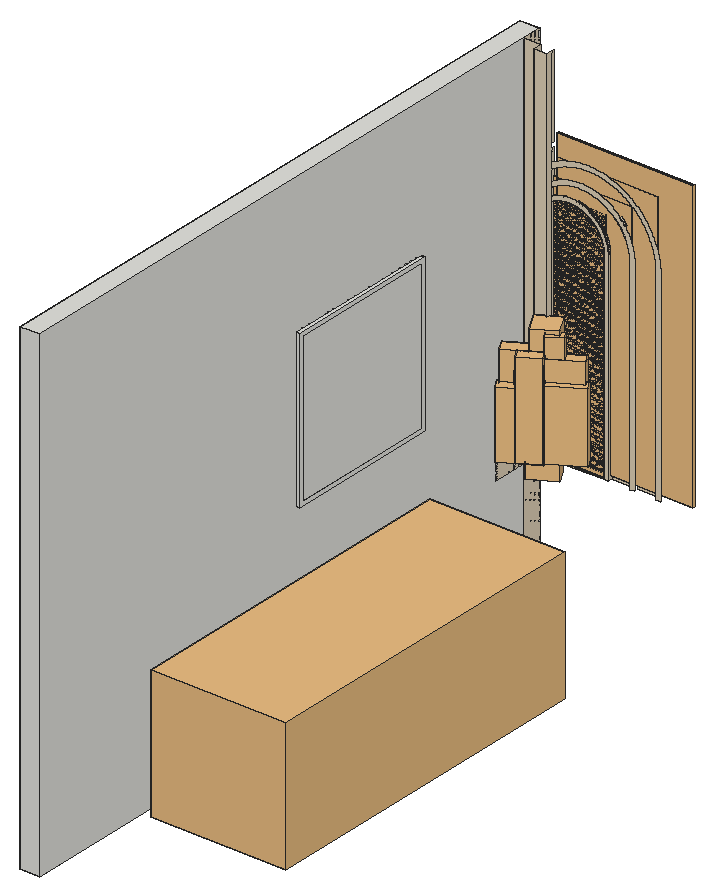
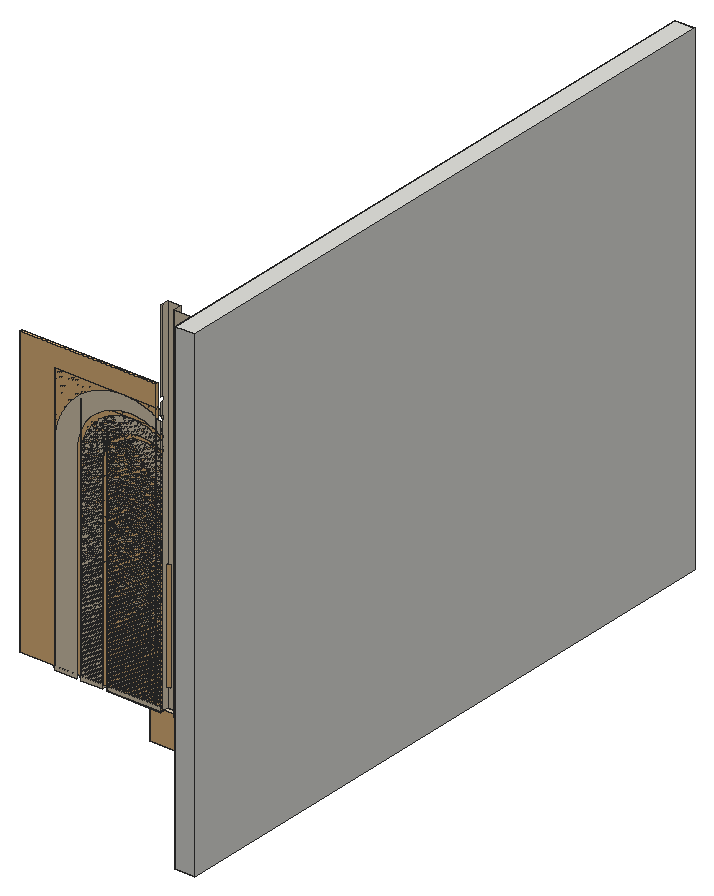
# SketchUp Ruby script. Lengths in inches.
U = 1.inch
M = Sketchup.active_model
def pt(a) = Geom::Point3d.new(a.map { |v| v * U })
def face(e, loops, mat)
  f = e.add_face(loops[0].map { |a| pt(a) })
  loops[1..].each { |l| e.add_face(l.map { |a| pt(a) }).erase! }
  f.material = f.back_material = mat if mat
  f
end
# faces: each face lists its corners as indices into pts; further lists are holes
def faces(e, pts, list, mat = nil) = list.each { |f| face(e, (f[0].is_a?(Array) ? f : [f]).map { |l| l.map { |i| pts[i] } }, mat) }
# xy, xz, yz: faces in a plane at the given z, y or x. An outline is a flat list of corners, or four numbers for a rectangle; further outlines are holes
def ring(l) = l.size == 4 ? [[l[0], l[1]], [l[2], l[1]], [l[2], l[3]], [l[0], l[3]]] : l.each_slice(2).to_a
def flat(e, list, mat, &to3) = list.each { |f| face(e, (f[0].is_a?(Array) ? f : [f]).map { |l| ring(l).map { |u, v| to3.(u, v) } }, mat) }
def xy(e, z, list, mat = nil) = flat(e, list, mat) { |x, y| [x, y, z] }
def xz(e, y, list, mat = nil) = flat(e, list, mat) { |x, z| [x, y, z] }
def yz(e, x, list, mat = nil) = flat(e, list, mat) { |y, z| [x, y, z] }
def lines(e, pts, list) = list.each { |a, b| e.add_line(pt(pts[a]), pt(pts[b])) }
# prism: a flat outline (further loops are holes) pulled along v
def prism(e, loops, v, mat = nil)
  f = face(e, loops, mat); d = Geom::Vector3d.new(v.map { |x| x * U })
  f.pushpull(f.normal.samedirection?(d) ? d.length : -d.length)
end
def box(e, o, s, mat = nil) = prism(e, [[o, [o[0] + s[0], o[1], o[2]], [o[0] + s[0], o[1] + s[1], o[2]], [o[0], o[1] + s[1], o[2]]]], [0, 0, s[2]], mat)
def at(x, y, z, deg = 0) = Geom::Transformation.translation(pt([x, y, z])) * Geom::Transformation.rotation(ORIGIN, Z_AXIS, deg.degrees)
def axes(o, x, y, z) = Geom::Transformation.new([*x, 0, *y, 0, *z, 0, *pt(o).to_a, 1])
def part(name) = M.definitions.add(name)
# library, detail: a bought-in or finely detailed component or shape, given as its bounding box
def library(name, o, s) = part(name).tap { |d| box(d.entities, o, s) }
def detail(e, o, s) = box(e.add_group.entities, o, s)
def put(e, d, t, mat = nil) = e.add_instance(d, t).tap { |i| i.material = mat if mat }
def group(e, t, mat = nil) = e.add_group.tap { |g| g.transformation = t; g.material = mat if mat }.entities
root = M.entities
M.materials.add("POT_TEXTURE_1").color = [172, 172, 172]
M.materials.add("Teddy_Brim").color = [225, 210, 185]
M.materials.add("soil1").color = [68, 55, 47]
c1 = library("Group\#92",[-662.41,217.3,320.04],[397.32,658.3,1732.06])
c2 = library("Group\#94",[-299.2,181.55,262.58],[360.65,735.71,1258.34])
c3 = library("Group\#89",[-1038.76,656.55,345.34],[733.18,460.51,2065.7])
c4 = library("Group\#87",[-445.29,890.31,329.28],[284.3,304.08,2023.29])
c5 = library("Group\#90",[-733.48,439.625,202.64],[456.28,533.12,1536.78])
c6 = library("Group\#93",[-455.56,899.32,410.78],[341.21,610.33,1581.5])
c7 = library("Group\#86",[-516.34,626.77,-4.5625],[517.73,515.95,418.98])
c8 = library("Group\#91",[-249.24,914.85,310.18],[345.55,647.95,1307.93])
c9 = library("Group\#88",[-277.97,488.68,287.26],[362.84,405.94,1768.54])
c10 = library("Group\#85",[-468.76,669.89,380.1875],[424.36,427.47,41.99])
c11 = part("Potted plant")
put(c11.entities,c1,at(1038.76,-181.55,4.5625))
put(c11.entities,c2,at(1038.76,-181.55,4.5625))
put(c11.entities,c3,at(1038.76,-181.55,4.5625))
put(c11.entities,c4,at(1038.76,-181.55,4.5625))
put(c11.entities,c5,at(1038.76,-181.55,4.5625))
put(c11.entities,c6,at(1038.76,-181.55,4.5625))
put(c11.entities,c7,at(1038.76,-181.55,4.5625),"POT_TEXTURE_1")
put(c11.entities,c8,at(1038.76,-181.55,4.5625))
put(c11.entities,c9,at(1038.76,-181.55,4.5625))
put(c11.entities,c10,at(1038.76,-181.55,4.5625),"soil1")
c12 = library("Group\#4",[0,0,0],[12.36,0.5,54.3])
c13 = library("Group\#3",[0,0,0],[18.36,0.5,57.11])
c14 = library("sofaD71839)",[0.35,-39.08,0.31],[80.46,34.29,30.24])
c15 = library("Group\#5",[0,0,0],[23.36,0.5,61.38])
c16 = library("Group\#155",[0,0,0],[31.36,0.5,66.36])
xy(root,34,[[8.5,137.5,11.5,137.6875],[8.5,137.6875,8.5,139.5,4.5,139.5,4.5,138.6875,11.5,138.6875,11.5,137.6875],[8.5,137.6875,11.5,138.6875],[11.5,138.5,23.86,138.6875],[23.86,138.5,24.86,138.6875],
  [11.5,138.6875,23.86,139.5]],"Teddy_Brim")
xy(root,88.29,[[15.22,138.5,15.4,139],[15.92,138.5,16.09,139]],"Teddy_Brim")
xy(root,88.3,[[15.57,138.5,15.74,139]],"Teddy_Brim")
xz(root,137.5,[[8.5,34,11.5,118]],"Teddy_Brim")
xz(root,138.5,[[11.5,33.76,11.5,34,24.86,34,24.86,80.61,24.85,80.8,24.85,80.98,24.83,81.17,24.82,81.35,24.8,81.54,24.77,81.72,24.75,81.9,24.72,82.08,24.68,82.27,24.64,82.45,24.6,82.625,24.55,82.81,24.5,82.98,24.45,83.16,24.39,83.34,24.33,83.51,24.26,83.68,24.19,83.86,24.12,84.03,24.05,84.19,23.97,84.36,23.88,84.53,23.8,84.69,23.71,84.85,23.61,85.01,23.52,85.17,23.42,85.33,23.3125,85.48,23.21,85.63,22.99,85.93,22.63,86.35,22.5,86.49,22.38,86.62,22.25,86.75,22.11,86.88,21.98,87.01,21.56,87.37,21.11,87.7,20.96,87.8,20.8,87.91,20.65,88,20.49,88.1,20.33,88.19,20.16,88.28,20,88.36,19.66,88.52,19.5,88.59,19.32,88.66,19.15,88.73,18.98,88.79,18.8,88.85,18.625,88.91,18.45,88.96,18.27,89.01,17.73,89.13,17.55,89.16,17.36,89.19,17.18,89.22,17,89.24,16.8125,89.26,16.63,89.27,16.44,89.28,16.26,89.28,16.07,89.29,15.89,89.28,15.7,89.28,15.52,89.27,15.33,89.26,14.97,89.22,14.78,89.19,14.42,89.13,14.06,89.05,13.875,89.01,13.7,88.96,13.52,88.91,13.34,88.85,13.17,88.79,12.99,88.73,12.48,88.52,12.3125,88.44,12.15,88.36,11.98,88.27,11.82,88.1875,11.66,88.09,11.5,88,11.5,87.17,11.6,87.23,11.75,87.3125,11.9,87.39,12.06,87.47,12.21,87.55,12.37,87.62,12.53,87.68,12.69,87.75,12.85,87.81,13.02,87.87,13.18,87.92,13.52,88.02,13.68,88.06,13.85,88.1,14.02,88.13,14.19,88.17,14.36,88.2,14.53,88.22,14.71,88.24,15.05,88.28,15.22,88.29,15.4,88.29,15.57,88.3,15.74,88.3,15.92,88.29,16.09,88.29,16.26,88.28,16.43,88.26,16.61,88.24,16.78,88.22,16.95,88.19,17.12,88.17,17.29,88.13,17.46,88.1,17.63,88.06,17.8,88.01,17.96,87.97,18.13,87.92,18.29,87.86,18.46,87.8,18.78,87.68,19.1,87.54,19.25,87.47,19.41,87.39,19.5625,87.31,19.71,87.22,19.86,87.14,20.01,87.05,20.16,86.95,20.3,86.86,20.58,86.66,20.86,86.44,21.12,86.22,21.25,86.1,21.5,85.86,21.62,85.74,21.73,85.61,21.85,85.48,21.96,85.35,22.07,85.21,22.18,85.08,22.28,84.9375,22.38,84.8,22.48,84.65,22.58,84.51,22.76,84.21,22.84,84.0625,22.93,83.91,23,83.76,23.08,83.6,23.22,83.28,23.29,83.125,23.35,82.96,23.47,82.64,23.57,82.3,23.61,82.14,23.73,81.63,23.79,81.29,23.83,80.95,23.85,80.77,23.86,80.6,23.86,34],[29.86,34,30.86,34,30.86,81.15,30.85,81.43,30.81,81.97,30.78,82.24,30.75,82.5,30.67,83.04,30.61,83.31,30.56,83.57,30.5,83.83,30.43,84.1,30.27,84.62,30.1875,84.87,30.1,85.13,29.9,85.63,29.79,85.88,29.68,86.125,29.56,86.37,29.43,86.61,29.31,86.85,29.17,87.09,28.89,87.55,28.74,87.77,28.58,88,28.42,88.21,28.26,88.43,27.92,88.85,27.74,89.05,27.56,89.26,26.99,89.83,26.79,90.02,26.58,90.19,26.375,90.37,26.17,90.54,25.95,90.71,25.73,90.87,25.29,91.17,25.06,91.32,24.83,91.46,24.59,91.6,24.36,91.73,24.12,91.85,23.87,91.97,23.63,92.09,23.38,92.2,23.13,92.3,22.875,92.4,22.62,92.49,22.37,92.58,21.85,92.74,21.59,92.81,21.32,92.87,21.06,92.93,20.79,92.98,20.53,93.03,19.99,93.11,19.72,93.13,19.45,93.16,19.18,93.18,18.91,93.1875,18.64,93.19,18.1,93.19,17.29,93.13,17.02,93.1,16.48,93.02,16.21,92.97,15.95,92.92,15.68,92.86,15.42,92.8,15.16,92.73,14.64,92.57,14.38,92.48,14.13,92.38,13.88,92.29,13.38,92.07,13.14,91.96,12.89,91.83,12.65,91.71,12.42,91.58,12.18,91.44,11.95,91.3,11.72,91.15,11.5,91,11.5,90.05,11.7,90.1875,11.92,90.33,12.36,90.59,12.58,90.71,12.8125,90.83,13.04,90.95,13.28,91.06,13.51,91.16,13.75,91.26,14.23,91.44,14.47,91.52,14.72,91.6,15.22,91.74,15.72,91.86,15.97,91.91,16.22,91.95,16.48,91.99,16.73,92.03,16.99,92.05,17.25,92.08,17.5,92.09,18.02,92.11,18.28,92.11,18.53,92.1,18.79,92.09,19.05,92.07,19.3,92.05,19.56,92.02,19.81,91.99,20.07,91.95,20.32,91.9,20.58,91.85,20.83,91.8,21.08,91.73,21.33,91.67,21.57,91.59,21.82,91.52,22.0625,91.43,22.3,91.34,22.54,91.25,22.78,91.15,23.02,91.04,23.48,90.82,23.71,90.7,23.93,90.57,24.15,90.45,24.375,90.31,24.59,90.17,24.8,90.03,25.01,89.88,25.22,89.72,25.42,89.57,25.625,89.4,25.82,89.24,26.01,89.07,26.39,88.71,26.57,88.53,26.74,88.34,26.92,88.15,27.09,87.96,27.41,87.56,27.57,87.35,27.72,87.14,27.86,86.93,28,86.71,28.14,86.5,28.27,86.27,28.4,86.05,28.64,85.59,28.86,85.13,28.96,84.89,29.05,84.65,29.15,84.41,29.23,84.17,29.3125,83.92,29.39,83.68,29.46,83.43,29.58,82.93,29.68,82.43,29.72,82.17,29.76,81.92,29.82,81.4,29.84,81.15,29.85,80.89,29.86,80.62],[35.86,34,36.86,34,36.86,80.61,36.85,80.97,36.83,81.67,36.8,82.03,36.77,82.38,36.73,82.73,36.68,83.08,36.56,83.78,36.49,84.125,36.41,84.47,36.33,84.8125,36.24,85.15,36.14,85.49,35.92,86.17,35.8,86.5,35.54,87.16,35.39,87.48,35.25,87.8,35.09,88.12,34.93,88.43,34.76,88.75,34.59,89.05,34.41,89.36,34.22,89.66,33.62,90.53,33.41,90.81,33.1875,91.09,32.96,91.37,32.74,91.64,32.26,92.16,31.51,92.91,31.24,93.14,30.98,93.375,30.71,93.6,30.15,94.04,29.86,94.25,29.28,94.65,28.98,94.84,28.68,95.02,28.375,95.2,27.75,95.54,27.43,95.69,27.12,95.84,26.79,95.99,26.47,96.13,26.14,96.26,25.81,96.38,25.47,96.5,25.14,96.61,24.46,96.81,24.11,96.89,23.77,96.98,23.42,97.05,23.08,97.12,22.73,97.17,22.38,97.23,21.68,97.31,21.32,97.34,20.97,97.36,20.62,97.375,20.26,97.38,19.91,97.38,19.56,97.37,19.2,97.36,18.15,97.27,17.45,97.17,17.1,97.11,16.4,96.97,16.06,96.88,15.72,96.8,15.04,96.6,14.7,96.48,14.37,96.37,13.71,96.11,13.38,95.97,13.0625,95.83,12.74,95.67,12.43,95.52,12.11,95.35,11.81,95.18,11.5,95,11.5,93.86,12.5,94.42,12.59,94.47,12.89,94.63,13.18,94.78,13.48,94.92,13.79,95.06,14.09,95.1875,14.4,95.3125,14.71,95.43,15.03,95.54,15.34,95.64,15.66,95.74,15.98,95.83,16.3,95.91,16.625,95.99,16.95,96.0625,17.28,96.125,17.6,96.18,17.93,96.23,18.59,96.31,18.93,96.34,19.26,96.36,19.92,96.38,20.25,96.38,20.59,96.375,20.92,96.36,21.25,96.34,21.58,96.3125,21.91,96.28,22.24,96.24,22.57,96.1875,22.9,96.13,23.23,96.07,23.55,96,24.2,95.84,24.52,95.75,24.84,95.65,25.15,95.55,25.47,95.44,26.09,95.2,26.39,95.07,26.7,94.9375,27,94.79,27.29,94.65,27.59,94.49,27.88,94.33,28.17,94.16,28.45,93.99,28.73,93.81,29.01,93.625,29.28,93.43,29.55,93.24,29.8125,93.04,30.07,92.83,30.33,92.61,30.58,92.4,30.82,92.17,31.07,91.94,31.3,91.71,31.76,91.23,32.2,90.73,32.41,90.47,32.61,90.21,32.8125,89.94,33.01,89.67,33.19,89.4,33.375,89.12,33.55,88.84,33.89,88.26,34.04,87.97,34.2,87.67,34.34,87.375,34.48,87.07,34.61,86.77,34.74,86.46,34.86,86.15,34.97,85.84,35.08,85.52,35.18,85.2,35.27,84.88,35.36,84.5625,35.4375,84.24,35.51,83.92,35.58,83.59,35.64,83.26,35.6875,82.93,35.73,82.6,35.77,82.27,35.83,81.61,35.84,81.28,35.86,80.95]],"Teddy_Brim")
xz(root,139.5,[[11.5,33.76,23.86,34,11.5,34],[4.5,34,8.5,118],[11.5,34,23.86,34,23.86,80.6,23.85,80.77,23.83,80.95,23.79,81.29,23.73,81.63,23.61,82.14,23.57,82.3,23.47,82.64,23.35,82.96,23.29,83.125,23.22,83.28,23.08,83.6,23,83.76,22.93,83.91,22.84,84.0625,22.76,84.21,22.58,84.51,22.48,84.65,22.38,84.8,22.28,84.9375,22.18,85.08,22.07,85.21,21.96,85.35,21.85,85.48,21.73,85.61,21.62,85.74,21.5,85.86,21.25,86.1,21.12,86.22,20.86,86.44,20.58,86.66,20.3,86.86,20.16,86.95,20.01,87.05,19.86,87.14,19.71,87.22,19.5625,87.31,19.41,87.39,19.25,87.47,19.1,87.54,18.78,87.68,18.46,87.8,18.29,87.86,18.13,87.92,17.96,87.97,17.8,88.01,17.63,88.06,17.46,88.1,17.29,88.13,17.12,88.17,16.95,88.19,16.78,88.22,16.61,88.24,16.43,88.26,16.26,88.28,16.09,88.29,15.92,88.29,15.74,88.3,15.57,88.3,15.4,88.29,15.22,88.29,15.05,88.28,14.71,88.24,14.53,88.22,14.36,88.2,14.19,88.17,14.02,88.13,13.85,88.1,13.68,88.06,13.52,88.02,13.18,87.92,13.02,87.87,12.85,87.81,12.69,87.75,12.53,87.68,12.37,87.62,12.21,87.55,12.06,87.47,11.9,87.39,11.75,87.3125,11.6,87.23,11.5,87.17],[24.86,34,29.86,34,29.86,80.62,29.85,80.89,29.84,81.15,29.82,81.4,29.76,81.92,29.72,82.17,29.68,82.43,29.58,82.93,29.46,83.43,29.39,83.68,29.3125,83.92,29.23,84.17,29.15,84.41,29.05,84.65,28.96,84.89,28.86,85.13,28.64,85.59,28.4,86.05,28.27,86.27,28.14,86.5,28,86.71,27.86,86.93,27.72,87.14,27.57,87.35,27.41,87.56,27.09,87.96,26.92,88.15,26.74,88.34,26.57,88.53,26.39,88.71,26.01,89.07,25.82,89.24,25.625,89.4,25.42,89.57,25.22,89.72,25.01,89.88,24.8,90.03,24.59,90.17,24.375,90.31,24.15,90.45,23.93,90.57,23.71,90.7,23.48,90.82,23.02,91.04,22.78,91.15,22.54,91.25,22.3,91.34,22.0625,91.43,21.82,91.52,21.57,91.59,21.33,91.67,21.08,91.73,20.83,91.8,20.58,91.85,20.32,91.9,20.07,91.95,19.81,91.99,19.56,92.02,19.3,92.05,19.05,92.07,18.79,92.09,18.53,92.1,18.28,92.11,18.02,92.11,17.5,92.09,17.25,92.08,16.99,92.05,16.73,92.03,16.48,91.99,16.22,91.95,15.97,91.91,15.72,91.86,15.22,91.74,14.72,91.6,14.47,91.52,14.23,91.44,13.75,91.26,13.51,91.16,13.28,91.06,13.04,90.95,12.8125,90.83,12.58,90.71,12.36,90.59,11.92,90.33,11.7,90.1875,11.5,90.05,11.5,88,11.66,88.09,11.82,88.1875,11.98,88.27,12.15,88.36,12.3125,88.44,12.48,88.52,12.99,88.73,13.17,88.79,13.34,88.85,13.52,88.91,13.7,88.96,13.875,89.01,14.06,89.05,14.42,89.13,14.78,89.19,14.97,89.22,15.33,89.26,15.52,89.27,15.7,89.28,15.89,89.28,16.07,89.29,16.26,89.28,16.44,89.28,16.63,89.27,16.8125,89.26,17,89.24,17.18,89.22,17.36,89.19,17.55,89.16,17.73,89.13,18.27,89.01,18.45,88.96,18.625,88.91,18.8,88.85,18.98,88.79,19.15,88.73,19.32,88.66,19.5,88.59,19.66,88.52,20,88.36,20.16,88.28,20.33,88.19,20.49,88.1,20.65,88,20.8,87.91,20.96,87.8,21.11,87.7,21.56,87.37,21.98,87.01,22.11,86.88,22.25,86.75,22.38,86.62,22.5,86.49,22.63,86.35,22.99,85.93,23.21,85.63,23.3125,85.48,23.42,85.33,23.52,85.17,23.61,85.01,23.71,84.85,23.8,84.69,23.88,84.53,23.97,84.36,24.05,84.19,24.12,84.03,24.19,83.86,24.26,83.68,24.33,83.51,24.39,83.34,24.45,83.16,24.5,82.98,24.55,82.81,24.6,82.625,24.64,82.45,24.68,82.27,24.72,82.08,24.75,81.9,24.77,81.72,24.8,81.54,24.82,81.35,24.83,81.17,24.85,80.98,24.85,80.8,24.86,80.61],[30.86,34,35.86,34,35.86,80.95,35.84,81.28,35.83,81.61,35.77,82.27,35.73,82.6,35.6875,82.93,35.64,83.26,35.58,83.59,35.51,83.92,35.4375,84.24,35.36,84.5625,35.27,84.88,35.18,85.2,35.08,85.52,34.97,85.84,34.86,86.15,34.74,86.46,34.61,86.77,34.48,87.07,34.34,87.375,34.2,87.67,34.04,87.97,33.89,88.26,33.55,88.84,33.375,89.12,33.19,89.4,33.01,89.67,32.8125,89.94,32.61,90.21,32.41,90.47,32.2,90.73,31.76,91.23,31.3,91.71,31.07,91.94,30.82,92.17,30.58,92.4,30.33,92.61,30.07,92.83,29.8125,93.04,29.55,93.24,29.28,93.43,29.01,93.625,28.73,93.81,28.45,93.99,28.17,94.16,27.88,94.33,27.59,94.49,27.29,94.65,27,94.79,26.7,94.9375,26.39,95.07,26.09,95.2,25.47,95.44,25.15,95.55,24.84,95.65,24.52,95.75,24.2,95.84,23.55,96,23.23,96.07,22.9,96.13,22.57,96.1875,22.24,96.24,21.91,96.28,21.58,96.3125,21.25,96.34,20.92,96.36,20.59,96.375,20.25,96.38,19.92,96.38,19.26,96.36,18.93,96.34,18.59,96.31,17.93,96.23,17.6,96.18,17.28,96.125,16.95,96.0625,16.625,95.99,16.3,95.91,15.98,95.83,15.66,95.74,15.34,95.64,15.03,95.54,14.71,95.43,14.4,95.3125,14.09,95.1875,13.79,95.06,13.48,94.92,13.18,94.78,12.89,94.63,12.59,94.47,12.5,94.42,11.5,93.86,11.5,91,11.72,91.15,11.95,91.3,12.18,91.44,12.42,91.58,12.65,91.71,12.89,91.83,13.14,91.96,13.38,92.07,13.88,92.29,14.13,92.38,14.38,92.48,14.64,92.57,15.16,92.73,15.42,92.8,15.68,92.86,15.95,92.92,16.21,92.97,16.48,93.02,17.02,93.1,17.29,93.13,18.1,93.19,18.64,93.19,18.91,93.1875,19.18,93.18,19.45,93.16,19.72,93.13,19.99,93.11,20.53,93.03,20.79,92.98,21.06,92.93,21.32,92.87,21.59,92.81,21.85,92.74,22.37,92.58,22.62,92.49,22.875,92.4,23.13,92.3,23.38,92.2,23.63,92.09,23.87,91.97,24.12,91.85,24.36,91.73,24.59,91.6,24.83,91.46,25.06,91.32,25.29,91.17,25.73,90.87,25.95,90.71,26.17,90.54,26.375,90.37,26.58,90.19,26.79,90.02,26.99,89.83,27.56,89.26,27.74,89.05,27.92,88.85,28.26,88.43,28.42,88.21,28.58,88,28.74,87.77,28.89,87.55,29.17,87.09,29.31,86.85,29.43,86.61,29.56,86.37,29.68,86.125,29.79,85.88,29.9,85.63,30.1,85.13,30.1875,84.87,30.27,84.62,30.43,84.1,30.5,83.83,30.56,83.57,30.61,83.31,30.67,83.04,30.75,82.5,30.78,82.24,30.81,81.97,30.85,81.43,30.86,81.15]],"Teddy_Brim")
yz(root,4.5,[[139.5,6,139.5,30,131.5,30,131.5,34,139.5,34,139.5,118,144,118,144,6]],"Teddy_Brim")
yz(root,8.5,[[137.5,34,139.5,118]],"Teddy_Brim")
yz(root,11.5,[[138.5,33.76,139.5,34],[137.5,34,138.9,34,138.9,87.17,138.5,87.17,138.5,88,138.9,88,138.9,90.05,138.5,90.05,138.5,91,138.9,91,138.9,93.86,138.5,93.86,138.5,95,138.9,95,138.9,97.85,138.5,97.85,138.5,99,138.9,99,138.9,118,137.5,118]],"Teddy_Brim")
yz(root,23.86,[[138.5,34,139,80.6]],"Teddy_Brim")
yz(root,24.85,[[138.5,80.8,139.5,80.98]],"Teddy_Brim")
yz(root,24.86,[[138.5,34,139.5,80.61]],"Teddy_Brim")
p = [[23.86,139.5,34],[11.5,139.5,33.76],[11.5,138.5,33.76],[23.86,138.5,34],[23.86,138.6875,34],[23.86,139,34],
  [23.85,138.5,80.77],[23.85,139,80.77],[23.86,139,80.6],[23.86,138.5,80.6],[24.86,139.5,80.61],[24.85,139.5,80.8],
  [24.85,138.5,80.8],[24.86,138.5,80.61],[23.83,138.5,80.95],[23.83,139,80.95],[23.81,138.5,81.12],[23.81,139,81.12],
  [24.85,139.5,80.98],[24.83,139.5,81.17],[24.83,138.5,81.17],[24.85,138.5,80.98],[23.79,138.5,81.29],[23.79,139,81.29],
  [24.82,139.5,81.35],[24.82,138.5,81.35],[23.76,138.5,81.46],[23.76,139,81.46],[24.8,139.5,81.54],[24.8,138.5,81.54],
  [23.73,138.5,81.63],[23.73,139,81.63],[24.77,139.5,81.72],[24.77,138.5,81.72],[23.69,138.5,81.8],[23.69,139,81.8],
  [24.75,139.5,81.9],[24.75,138.5,81.9],[23.65,138.5,81.97],[23.65,139,81.97],[24.72,139.5,82.08],[24.72,138.5,82.08],
  [23.61,138.5,82.14],[23.61,139,82.14],[23.57,138.5,82.3],[23.57,139,82.3],[24.68,139.5,82.27],[24.68,138.5,82.27],
  [23.52,138.5,82.47],[23.52,139,82.47],[24.64,139.5,82.45],[24.64,138.5,82.45],[24.6,139.5,82.625],[24.6,138.5,82.625],
  [23.47,138.5,82.64],[23.47,139,82.64],[23.41,138.5,82.8],[23.41,139,82.8],[24.55,139.5,82.81],[24.55,138.5,82.81],
  [23.35,138.5,82.96],[23.35,139,82.96],[24.5,139.5,82.98],[24.5,138.5,82.98],[23.29,138.5,83.125],[23.29,139,83.125],
  [24.45,139.5,83.16],[24.45,138.5,83.16],[23.22,138.5,83.28],[23.22,139,83.28],[24.39,139.5,83.34],[24.39,138.5,83.34],
  [23.15,138.5,83.44],[23.15,139,83.44],[24.33,139.5,83.51],[24.33,138.5,83.51],[23.08,138.5,83.6],[23.08,139,83.6],
  [24.26,139.5,83.68],[24.26,138.5,83.68],[23,138.5,83.76],[23,139,83.76],[24.19,139.5,83.86],[24.19,138.5,83.86],
  [22.93,138.5,83.91],[22.93,139,83.91],[22.84,138.5,84.0625],[22.84,139,84.0625],[24.12,139.5,84.03],[24.12,138.5,84.03],
  [24.05,139.5,84.19],[24.05,138.5,84.19],[22.76,138.5,84.21],[22.76,139,84.21],[22.67,138.5,84.36],[22.67,139,84.36],
  [23.97,139.5,84.36],[23.97,138.5,84.36],[22.58,138.5,84.51],[22.58,139,84.51],[23.88,139.5,84.53],[23.88,138.5,84.53],
  [22.48,138.5,84.65],[22.48,139,84.65],[23.8,139.5,84.69],[23.8,138.5,84.69],[22.38,138.5,84.8],[22.38,139,84.8],
  [23.71,139.5,84.85],[23.71,138.5,84.85],[22.28,138.5,84.9375],[22.28,139,84.9375],[22.18,138.5,85.08],[22.18,139,85.08],
  [23.61,139.5,85.01],[23.61,138.5,85.01],[23.52,139.5,85.17],[23.52,138.5,85.17],[22.07,138.5,85.21],[22.07,139,85.21],
  [21.96,138.5,85.35],[21.96,139,85.35],[23.42,139.5,85.33],[23.42,138.5,85.33],[21.85,138.5,85.48],[21.85,139,85.48],
  [23.3125,139.5,85.48],[23.3125,138.5,85.48],[28.64,138.5,85.59],[28.64,139,85.59],[28.75,139,85.36],[28.75,138.5,85.36],
  [21.73,138.5,85.61],[21.73,139,85.61],[23.21,139.5,85.63],[23.21,138.5,85.63],[21.62,138.5,85.74],[21.62,139,85.74],
  [23.1,139.5,85.78],[23.1,138.5,85.78],[28.52,138.5,85.82],[28.52,139,85.82],[21.5,138.5,85.86],[21.5,139,85.86],
  [22.99,139.5,85.93],[22.99,138.5,85.93],[28.4,138.5,86.05],[28.4,139,86.05],[21.375,138.5,85.98],[21.375,139,85.98],
  [22.87,139.5,86.07],[22.87,138.5,86.07],[21.25,138.5,86.1],[21.25,139,86.1],[21.12,138.5,86.22],[21.12,139,86.22],
  [22.75,139.5,86.21],[22.75,138.5,86.21],[28.27,138.5,86.27],[28.27,139,86.27],[20.99,138.5,86.33],[20.99,139,86.33],
  [22.63,139.5,86.35],[22.63,138.5,86.35],[20.86,138.5,86.44],[20.86,139,86.44],[28.14,138.5,86.5],[28.14,139,86.5],
  [20.72,138.5,86.55],[20.72,139,86.55],[22.5,139.5,86.49],[22.5,138.5,86.49],[22.38,139.5,86.62],[22.38,138.5,86.62],
  [28,138.5,86.71],[28,139,86.71],[20.58,138.5,86.66],[20.58,139,86.66],[22.25,139.5,86.75],[22.25,138.5,86.75],
  [20.44,138.5,86.76],[20.44,139,86.76],[27.86,138.5,86.93],[27.86,139,86.93],[20.3,138.5,86.86],[20.3,139,86.86],
  [22.11,139.5,86.88],[22.11,138.5,86.88],[20.16,138.5,86.95],[20.16,139,86.95],[21.98,139.5,87.01],[21.98,138.5,87.01],
  [27.72,138.5,87.14],[27.72,139,87.14],[19.86,138.5,87.14],[19.86,139,87.14],[20.01,139,87.05],[20.01,138.5,87.05],
  [21.84,139.5,87.13],[21.84,138.5,87.13],[19.71,138.5,87.22],[19.71,139,87.22],[21.7,139.5,87.25],[21.7,138.5,87.25],
  [27.57,138.5,87.35],[27.57,139,87.35],[11.5,138.9,87.17],[11.5,139,87.17],[11.6,139,87.23],[11.6,138.5,87.23],
  [11.5,138.5,87.17],[11.75,139,87.3125],[11.75,138.5,87.3125],[19.5625,138.5,87.31],[19.5625,139,87.31],[11.9,139,87.39],
  [11.9,138.5,87.39],[19.41,138.5,87.39],[19.41,139,87.39],[21.56,139.5,87.37],[21.56,138.5,87.37],[12.06,139,87.47],
  [12.06,138.5,87.47],[19.25,138.5,87.47],[19.25,139,87.47],[21.41,139.5,87.48],[21.41,138.5,87.48],[27.41,138.5,87.56],
  [27.41,139,87.56],[12.21,139,87.55],[12.21,138.5,87.55],[12.37,139,87.62],[12.37,138.5,87.62],[18.94,138.5,87.61],
  [18.94,139,87.61],[19.1,139,87.54],[19.1,138.5,87.54],[21.26,139.5,87.59],[21.26,138.5,87.59],[12.53,139,87.68],
  [12.53,138.5,87.68],[18.78,138.5,87.68],[18.78,139,87.68],[21.11,139.5,87.7],[21.11,138.5,87.7],[27.25,138.5,87.76],
  [27.25,139,87.76],[12.69,139,87.75],[12.69,138.5,87.75],[12.85,139,87.81],[12.85,138.5,87.81],[18.46,138.5,87.8],
  [18.46,139,87.8],[18.62,139,87.74],[18.62,138.5,87.74],[20.96,139.5,87.8],[20.96,138.5,87.8],[13.02,139,87.87],
  [13.02,138.5,87.87],[18.29,138.5,87.86],[18.29,139,87.86],[20.8,139.5,87.91],[20.8,138.5,87.91],[27.09,138.5,87.96],
  [27.09,139,87.96],[28.74,139.5,87.77],[28.58,139.5,88],[28.58,138.5,88],[28.74,138.5,87.77],[13.18,139,87.92],
  [13.18,138.5,87.92],[13.35,139,87.97],[13.35,138.5,87.97],[17.96,138.5,87.97],[17.96,139,87.97],[18.13,139,87.92],
  [18.13,138.5,87.92],[20.65,139.5,88],[20.65,138.5,88],[11.66,139.5,88.09],[11.5,139.5,88],[11.5,138.9,88],
  [11.5,138.5,88],[11.66,138.5,88.09],[13.52,139,88.02],[13.52,138.5,88.02],[13.68,139,88.06],[13.68,138.5,88.06],
  [17.63,138.5,88.06],[17.63,139,88.06],[17.8,139,88.01],[17.8,138.5,88.01],[20.49,139.5,88.1],[20.49,138.5,88.1],
  [26.92,138.5,88.15],[26.92,139,88.15],[28.42,139.5,88.21],[28.42,138.5,88.21],[11.82,139.5,88.1875],[11.82,138.5,88.1875],
  [13.85,139,88.1],[13.85,138.5,88.1],[14.02,139,88.13],[14.02,138.5,88.13],[14.19,139,88.17],[14.19,138.5,88.17],
  [17.12,138.5,88.17],[17.12,139,88.17],[17.29,139,88.13],[17.29,138.5,88.13],[17.46,139,88.1],[17.46,138.5,88.1],
  [20.33,139.5,88.19],[20.33,138.5,88.19],[11.98,139.5,88.27],[11.98,138.5,88.27],[14.36,139,88.2],[14.36,138.5,88.2],
  [14.53,139,88.22],[14.53,138.5,88.22],[14.71,139,88.24],[14.71,138.5,88.24],[14.88,139,88.26],[14.88,138.5,88.26],
  [16.43,138.5,88.26],[16.43,139,88.26],[16.61,139,88.24],[16.61,138.5,88.24],[16.78,139,88.22],[16.78,138.5,88.22],
  [16.95,139,88.19],[16.95,138.5,88.19],[20.16,139.5,88.28],[20.16,138.5,88.28],[26.74,138.5,88.34],[26.74,139,88.34],
  [28.26,139.5,88.43],[28.26,138.5,88.43],[12.15,139.5,88.36],[12.15,138.5,88.36],[15.05,139,88.28],[15.05,138.5,88.28],
  [15.22,139,88.29],[15.22,138.5,88.29],[15.4,138.5,88.29],[15.4,139,88.29],[15.57,139,88.3],[15.57,138.5,88.3],
  [15.74,138.5,88.3],[15.74,139,88.3],[15.92,139,88.29],[15.92,138.5,88.29],[16.09,138.5,88.29],[16.09,139,88.29],
  [16.26,139,88.28],[16.26,138.5,88.28],[20,139.5,88.36],[20,138.5,88.36],[26.57,138.5,88.53],[26.57,139,88.53],
  [12.3125,139.5,88.44],[12.3125,138.5,88.44],[12.48,139.5,88.52],[12.48,138.5,88.52],[19.83,139.5,88.44],[19.66,139.5,88.52],
  [19.66,138.5,88.52],[19.83,138.5,88.44],[28.09,139.5,88.64],[28.09,138.5,88.64],[12.65,139.5,88.59],[12.65,138.5,88.59],
  [19.5,139.5,88.59],[19.5,138.5,88.59],[26.39,138.5,88.71],[26.39,139,88.71],[12.82,139.5,88.66],[12.82,138.5,88.66],
  [19.32,139.5,88.66],[19.32,138.5,88.66],[27.92,139.5,88.85],[27.92,138.5,88.85],[12.99,139.5,88.73],[12.99,138.5,88.73],
  [13.17,139.5,88.79],[13.17,138.5,88.79],[19.15,139.5,88.73],[18.98,139.5,88.79],[18.98,138.5,88.79],[19.15,138.5,88.73],
  [26.2,138.5,88.89],[26.2,139,88.89],[13.34,139.5,88.85],[13.34,138.5,88.85],[18.8,139.5,88.85],[18.8,138.5,88.85],
  [13.52,139.5,88.91],[13.52,138.5,88.91],[13.7,139.5,88.96],[13.7,138.5,88.96],[18.625,139.5,88.91],[18.45,139.5,88.96],
  [18.45,138.5,88.96],[18.625,138.5,88.91],[26.01,138.5,89.07],[26.01,139,89.07],[27.74,139.5,89.05],[27.74,138.5,89.05],
  [13.875,139.5,89.01],[13.875,138.5,89.01],[14.06,139.5,89.05],[14.06,138.5,89.05],[18.27,139.5,89.01],[18.09,139.5,89.05],
  [18.09,138.5,89.05],[18.27,138.5,89.01],[14.24,139.5,89.09],[14.24,138.5,89.09],[14.42,139.5,89.13],[14.42,138.5,89.13],
  [14.6,139.5,89.16],[14.6,138.5,89.16],[17.73,139.5,89.13],[17.55,139.5,89.16],[17.55,138.5,89.16],[17.73,138.5,89.13],
  [17.91,139.5,89.09],[17.91,138.5,89.09],[25.82,138.5,89.24],[25.82,139,89.24],[27.56,139.5,89.26],[27.56,138.5,89.26]]
faces(root,p,[[0,1,2,3,4,5],[6,7,8,9],[10,11,12,13],[14,15,7,6],[16,17,15,14],[18,19,20,21],[22,23,17,16],[19,24,25,20],
  [26,27,23,22],[24,28,29,25],[30,31,27,26],[28,32,33,29],[34,35,31,30],[32,36,37,33],[38,39,35,34],[36,40,41,37],
  [42,43,39,38],[44,45,43,42],[40,46,47,41],[48,49,45,44],[46,50,51,47],[50,52,53,51],[54,55,49,48],[56,57,55,54],
  [52,58,59,53],[60,61,57,56],[58,62,63,59],[64,65,61,60],[62,66,67,63],[68,69,65,64],[66,70,71,67],[72,73,69,68],
  [70,74,75,71],[76,77,73,72],[74,78,79,75],[80,81,77,76],[78,82,83,79],[84,85,81,80],[86,87,85,84],[82,88,89,83],
  [88,90,91,89],[92,93,87,86],[94,95,93,92],[90,96,97,91],[98,99,95,94],[96,100,101,97],[102,103,99,98],[100,104,105,101],
  [106,107,103,102],[104,108,109,105],[110,111,107,106],[112,113,111,110],[108,114,115,109],[114,116,117,115],[118,119,113,112],[120,121,119,118],
  [116,122,123,117],[124,125,121,120],[122,126,127,123],[128,129,130,131],[132,133,125,124],[126,134,135,127],[136,137,133,132],[134,138,139,135],
  [140,141,129,128],[142,143,137,136],[138,144,145,139],[146,147,141,140],[148,149,143,142],[144,150,151,145],[152,153,149,148],[154,155,153,152],
  [150,156,157,151],[158,159,147,146],[160,161,155,154],[156,162,163,157],[164,165,161,160],[166,167,159,158],[168,169,165,164],[162,170,171,163],
  [170,172,173,171],[174,175,167,166],[176,177,169,168],[172,178,179,173],[180,181,177,176],[182,183,175,174],[184,185,181,180],[178,186,187,179],
  [188,189,185,184],[186,190,191,187],[192,193,183,182],[194,195,196,197],[197,196,189,188],[190,198,199,191],[200,201,195,194],[198,202,203,199],
  [204,205,193,192],[206,207,208,209,210],[209,208,211,212],[213,214,201,200],[212,211,215,216],[217,218,214,213],[202,219,220,203],[216,215,221,222],
  [223,224,218,217],[219,225,226,220],[227,228,205,204],[222,221,229,230],[230,229,231,232],[233,234,235,236],[236,235,224,223],[225,237,238,226],
  [232,231,239,240],[241,242,234,233],[237,243,244,238],[245,246,228,227],[240,239,247,248],[248,247,249,250],[251,252,253,254],[254,253,242,241],
  [243,255,256,244],[250,249,257,258],[259,260,252,251],[255,261,262,256],[263,264,246,245],[265,266,267,268],[258,257,269,270],[270,269,271,272],
  [273,274,275,276],[276,275,260,259],[261,277,278,262],[279,280,281,282,283],[272,271,284,285],[285,284,286,287],[288,289,290,291],[291,290,274,273],
  [277,292,293,278],[294,295,264,263],[266,296,297,267],[298,279,283,299],[287,286,300,301],[301,300,302,303],[303,302,304,305],[306,307,308,309],
  [309,308,310,311],[311,310,289,288],[292,312,313,293],[314,298,299,315],[305,304,316,317],[317,316,318,319],[319,318,320,321],[321,320,322,323],
  [324,325,326,327],[327,326,328,329],[329,328,330,331],[331,330,307,306],[312,332,333,313],[334,335,295,294],[296,336,337,297],[338,314,315,339],
  [323,322,340,341],[341,340,342,343],[344,345,346,347],[348,349,350,351],[352,353,354,355],[355,354,325,324],[332,356,357,333],[358,359,335,334],
  [360,338,339,361],[362,360,361,363],[364,365,366,367],[356,364,367,357],[336,368,369,337],[370,362,363,371],[365,372,373,366],[374,375,359,358],
  [376,370,371,377],[372,378,379,373],[368,380,381,369],[382,376,377,383],[384,382,383,385],[386,387,388,389],[378,386,389,379],[390,391,375,374],
  [392,384,385,393],[387,394,395,388],[396,392,393,397],[398,396,397,399],[400,401,402,403],[394,400,403,395],[404,405,391,390],[380,406,407,381],
  [408,398,399,409],[410,408,409,411],[412,413,414,415],[401,412,415,402],[416,410,411,417],[418,416,417,419],[420,418,419,421],[422,423,424,425],
  [426,422,425,427],[413,426,427,414],[428,429,405,404],[406,430,431,407]],"Teddy_Brim")
g1 = group(root,at(0,0,6))
box(g1,[0,0,0],[4.5,144,112])
g2 = group(root,at(4.5,73.75,50.09))
xy(g2,0,[[0,0,0.98,36]])
xy(g2,0.79,[[0.67,0.79,0.98,35.21]])
xy(g2,35.21,[[0.67,0.79,0.98,35.21]])
xy(g2,36,[[0,0,0.98,36]])
xz(g2,0,[[0,0,0.98,36]])
xz(g2,0.79,[[0.67,0.79,0.98,35.21]])
xz(g2,35.21,[[0.67,0.79,0.98,35.21]])
xz(g2,36,[[0,0,0.98,36]])
yz(g2,0,[[0,0,36,36]])
yz(g2,0.67,[[0.79,0.79,35.21,35.21]])
yz(g2,0.98,[[[0,0,36,36],[0.79,0.79,35.21,35.21]]])
g3 = group(root,at(11.5,138.9,34),"Teddy_Brim")
yz(g3,0,[[0,0,0.6,53.17],[0,54,0.6,56.05],[0,57,0.6,59.86],[0,61,0.6,63.85],[0,65,0.6,84]])
put(root,c11,axes([4.03,133.62,34],[0.00376,-0.00652,0],[0.01068,0.00617,0],[0,0,0.01233]))
put(root,c12,at(11.5,139,34),"Teddy_Brim")
put(root,c13,at(11.5,139,35),"Teddy_Brim")
put(root,c14,axes([1.96,29.3,5.69],[0,1,0],[-0.91,0,0],[0,0,1]))
put(root,c15,at(12.5,139,35),"Teddy_Brim")
put(root,c16,at(12.5,139,35),"Teddy_Brim")
